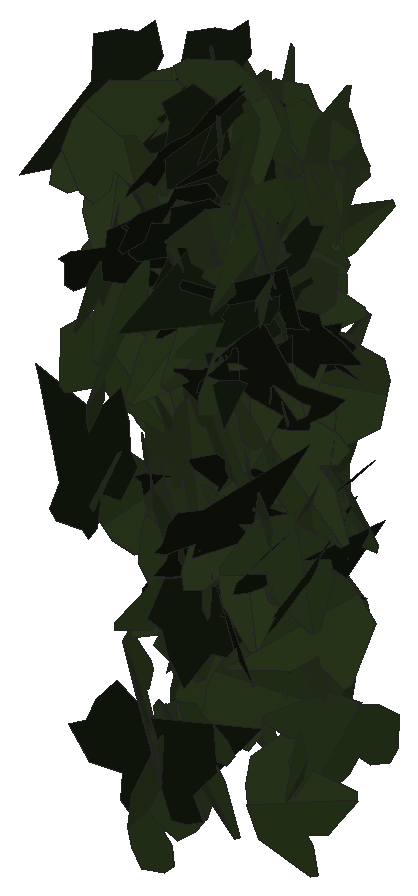
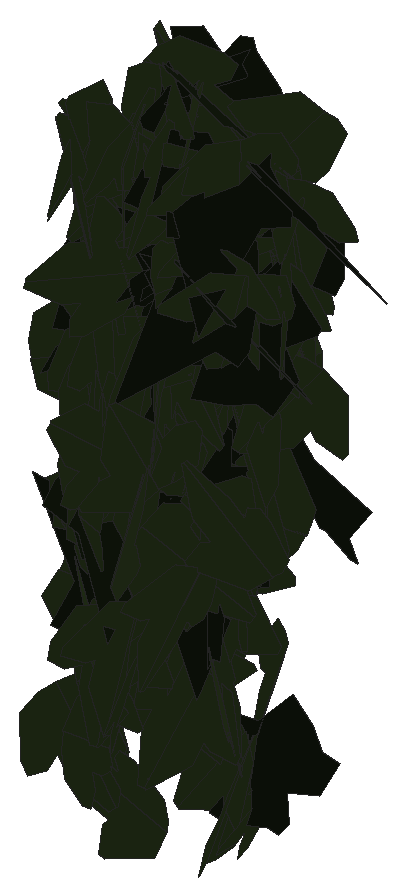
# SketchUp Ruby script. Lengths in inches.
U = 1.inch
M = Sketchup.active_model
def pt(a) = Geom::Point3d.new(a.map { |v| v * U })
def face(e, loops, mat)
  f = e.add_face(loops[0].map { |a| pt(a) })
  loops[1..].each { |l| e.add_face(l.map { |a| pt(a) }).erase! }
  f.material = f.back_material = mat if mat
  f
end
# faces: each face lists its corners as indices into pts; further lists are holes
def faces(e, pts, list, mat = nil) = list.each { |f| face(e, (f[0].is_a?(Array) ? f : [f]).map { |l| l.map { |i| pts[i] } }, mat) }
# xy, xz, yz: faces in a plane at the given z, y or x. An outline is a flat list of corners, or four numbers for a rectangle; further outlines are holes
def ring(l) = l.size == 4 ? [[l[0], l[1]], [l[2], l[1]], [l[2], l[3]], [l[0], l[3]]] : l.each_slice(2).to_a
def flat(e, list, mat, &to3) = list.each { |f| face(e, (f[0].is_a?(Array) ? f : [f]).map { |l| ring(l).map { |u, v| to3.(u, v) } }, mat) }
def xy(e, z, list, mat = nil) = flat(e, list, mat) { |x, y| [x, y, z] }
def xz(e, y, list, mat = nil) = flat(e, list, mat) { |x, z| [x, y, z] }
def yz(e, x, list, mat = nil) = flat(e, list, mat) { |y, z| [x, y, z] }
def lines(e, pts, list) = list.each { |a, b| e.add_line(pt(pts[a]), pt(pts[b])) }
# prism: a flat outline (further loops are holes) pulled along v
def prism(e, loops, v, mat = nil)
  f = face(e, loops, mat); d = Geom::Vector3d.new(v.map { |x| x * U })
  f.pushpull(f.normal.samedirection?(d) ? d.length : -d.length)
end
def box(e, o, s, mat = nil) = prism(e, [[o, [o[0] + s[0], o[1], o[2]], [o[0] + s[0], o[1] + s[1], o[2]], [o[0], o[1] + s[1], o[2]]]], [0, 0, s[2]], mat)
def at(x, y, z, deg = 0) = Geom::Transformation.translation(pt([x, y, z])) * Geom::Transformation.rotation(ORIGIN, Z_AXIS, deg.degrees)
def axes(o, x, y, z) = Geom::Transformation.new([*x, 0, *y, 0, *z, 0, *pt(o).to_a, 1])
def part(name) = M.definitions.add(name)
# library, detail: a bought-in or finely detailed component or shape, given as its bounding box
def library(name, o, s) = part(name).tap { |d| box(d.entities, o, s) }
def detail(e, o, s) = box(e.add_group.entities, o, s)
def put(e, d, t, mat = nil) = e.add_instance(d, t).tap { |i| i.material = mat if mat }
def group(e, t, mat = nil) = e.add_group.tap { |g| g.transformation = t; g.material = mat if mat }.entities
root = M.entities
M.materials.add("efeu1").color = [18, 25, 13]
M.materials.add("efeu2").color = [43, 57, 29]
c1 = part("ivyleaf_9")
p = [[1.54,2.16,1.25],[1.36,2.04,1.19],[-0.21,0.99,0.68],[-0.71,1.11,0.82],[-0.85,0.86,0.67],[-0.8,0.17,0.21],
  [-0.9,-0.01,0.1],[-0.67,-0.16,-0.02],[-0.08,-0.08,-0.05],[-0.03,-0.6,-0.4],[0.65,-0.88,-0.66],[0.83,-0.6,-0.49],
  [1.29,-0.42,-0.43],[1.8125,-0.07,-0.26],[1.21,0.44,0.15]]
faces(c1.entities,p,[[0,1,2,3,4,5,6,7,8,9,10,11,12,13,14]],"efeu1")
c2 = part("ivyleaf_10")
p = [[0,0.5,-0.03],[-0.0625,2.02,-0.43],[-0.19,2.01,-0.46],[-0.54,1.05,-0.29],[-0.52,0.625,-0.18],[-0.83,0.76,-0.28],
  [-1.16,0.64,-0.33],[-1.15,0.33,-0.24],[-0.77,-0.39,0.02],[-0.3,-0.51,0.16],[0.04,-0.48,0.23],[-0.02,2.01,-0.4375],
  [-0.06,2.01,-0.43],[0.04,-0.49,0.23],[0.67,-0.49,0.14],[1.38,0.36,-0.2],[1.375,0.51,-0.24],[0.81,0.65,-0.19],
  [0.62,0.59,-0.15],[0.6,1.09,-0.28],[0.5,1.23,-0.31]]
faces(c2.entities,p,[[0,1,2,3,4,5,6,7,8,9,10],[11,12,0,13,14,15,16,17,18,19,20]],"efeu2")
put(root,c1,axes([53.01,224.28,213.86],[-0.08194,0.49287,-0.01911],[0.00066,-0.01926,-0.49963],[-0.49324,-0.08191,0.00251]))
put(root,c2,axes([53.49,224.47,213.82],[0.29891,-0.37756,-0.13453],[-0.0781,0.10975,-0.48151],[0.39313,0.30888,0.00664]))
put(root,c2,axes([53.17,224.42,212.98],[-0.47923,-0.13524,-0.04522],[0.04223,0.01686,-0.49793],[0.13621,-0.48107,-0.00474]))
put(root,c1,axes([52.24,224.17,212.53],[0.31543,0.37494,0.09961],[0.06207,0.07795,-0.48997],[-0.38295,0.32147,0.00263]))
put(root,c2,axes([52.11,224.1875,211.125],[0.20626,-0.0813,0.44816],[-0.28646,0.35934,0.19702],[-0.35412,-0.33803,0.10166]))
put(root,c2,axes([52.12,224.58,213.11],[-0.31863,0.21038,-0.32282],[0.27616,-0.16744,-0.3817],[-0.26871,-0.42155,-0.00949]))
put(root,c2,axes([53.54,224.875,212.99],[0.00931,-0.29036,0.40695],[0.04826,-0.40459,-0.28978],[0.49758,0.04467,0.02049]))
put(root,c2,axes([52.0625,224.58,212.13],[0.44448,-0.22083,-0.06058],[-0.0461,0.04328,-0.49599],[0.2243,0.4465,0.01812]))
put(root,c2,axes([53.64,224.52,212.875],[0.3422,-0.33023,-0.15444],[-0.09926,0.11941,-0.47528],[0.35078,0.35594,0.01617]))
put(root,c1,axes([52.86,224.23,213.17],[0.13472,0.46802,0.11315],[0.03132,0.10873,-0.48703],[-0.48049,0.13832,-0.00002]))
put(root,c2,axes([53.26,224.81,212],[-0.22024,-0.24089,0.37877],[-0.18429,-0.33618,-0.32097],[0.4093,-0.28099,0.0593]))
put(root,c2,axes([53.59,224.49,213.13],[-0.30366,0.39692,0.01568],[-0.01009,0.01203,-0.49975],[-0.3971,-0.30383,0.0007]))
put(root,c1,axes([53,224.46,209.82],[0.24907,0.43347,0.00838],[-0.0061,-0.00616,0.49992],[0.4335,-0.24914,0.00222]))
put(root,c1,axes([53.27,224.6875,211.9],[0.494,0.07725,-0.00036],[-0.00038,0.00479,0.49998],[0.07725,-0.49397,0.00479]))
put(root,c1,axes([52.83,224.3125,212.89],[0.38483,0.31697,0.03793],[0.02521,0.02905,-0.49852],[-0.31824,0.3856,0.00638]))
put(root,c1,axes([53.42,224.87,212.58],[-0.42674,-0.15396,0.21021],[-0.1897,-0.09295,-0.45318],[0.17863,-0.46654,0.02092]))
put(root,c2,axes([52.18,224.59,208.21],[-0.29106,0.39887,-0.07866],[0.04703,-0.06305,-0.49377],[-0.40382,-0.29483,-0.00081]))
put(root,c2,axes([51.88,224.68,213.07],[0.49749,0.03328,0.03743],[0.03738,0.00194,-0.4986],[-0.03333,0.49889,-0.00056]))
put(root,c2,axes([52.03,224.375,213.56],[0.17565,0.3024,0.35735],[0.14418,0.32818,-0.34858],[-0.44537,0.2255,0.0281]))
put(root,c1,axes([51.91,224.42,209.96],[-0.05106,0.12132,0.48236],[-0.2897,0.38691,-0.12798],[-0.40431,-0.29255,0.03079]))
put(root,c2,axes([51.97,224.48,212.25],[0.05305,-0.37741,-0.32364],[-0.0349,0.32185,-0.38104],[0.49595,0.06302,0.0078]))
put(root,c1,axes([53.73,224.56,212.55],[-0.28381,0.35846,0.20238],[-0.2025,0.09244,-0.44772],[-0.35839,-0.3361,0.09271]))
put(root,c2,axes([53.65,224.83,212.46],[-0.2618,-0.37422,0.20353],[-0.11137,-0.17045,-0.45666],[0.41117,-0.28444,0.00589]))
put(root,c1,axes([53.21,224.81,211.06],[0.47177,0.10045,0.13169],[-0.12898,-0.02657,0.48235],[0.1039,-0.48908,0.00084]))
put(root,c2,axes([52.72,224.7,209.11],[-0.27081,-0.41819,-0.04217],[0.02998,0.03081,-0.49815],[0.41924,-0.27234,0.00839]))
put(root,c2,axes([52.9375,224.6875,211.05],[-0.45123,0.17443,-0.12635],[0.11304,-0.05787,-0.4836],[-0.18334,-0.465,0.01279]))
put(root,c2,axes([53.17,224.98,213.5],[0.16317,-0.39651,0.25721],[0.08733,-0.24212,-0.42866],[0.46449,0.18481,-0.00976]))
put(root,c2,axes([53.5,224.69,212.08],[-0.34925,0.18892,-0.30386],[-0.28043,0.11919,0.39642],[0.22222,0.44733,0.0227]))
put(root,c2,axes([52.4375,224.58,209.99],[-0.34802,0.20839,0.29233],[-0.26084,0.13298,-0.40532],[-0.24667,-0.43462,0.01615]))
put(root,c2,axes([53.26,224.84,211.88],[-0.15431,-0.47253,0.0539],[-0.00488,-0.05509,-0.49693],[0.47557,-0.15389,0.01239]))
put(root,c2,axes([51.73,224.76,211.22],[-0.38038,-0.133,-0.29601],[0.3159,-0.04738,-0.38465],[0.07426,-0.47965,0.12007]))
put(root,c2,axes([52.65,224.79,210.62],[-0.07809,0.48217,-0.10686],[0.01846,-0.10526,-0.48845],[-0.49352,-0.08023,-0.00136]))
put(root,c2,axes([52.85,224.68,212.46],[-0.42716,0.25307,0.05904],[-0.05057,0.03048,-0.4965],[-0.2549,-0.43015,-0.00044]))
put(root,c1,axes([51.98,224.74,207.09],[0.01906,0.00281,0.49963],[0.475,-0.15517,-0.01725],[0.15496,0.4753,-0.00858]))
put(root,c2,axes([53.13,224.84,213.93],[0.3117,-0.00481,-0.39092],[-0.39046,0.02115,-0.31159],[0.01953,0.49953,0.00943]))
put(root,c2,axes([52.72,224.92,212.78],[0.39517,-0.30034,0.06033],[0.04868,-0.03566,-0.49635],[0.30245,0.39815,0.00106]))
put(root,c2,axes([52.46,224.79,209.88],[-0.49592,-0.00803,-0.06327],[0.06366,-0.03258,-0.49486],[0.00382,-0.49887,0.03334]))
put(root,c1,axes([52.92,224.83,213.84],[0.10067,-0.42668,-0.24043],[-0.05798,0.23335,-0.43839],[0.48632,0.11615,-0.0025]))
put(root,c2,axes([53.3,224.79,211.54],[0.18564,0.46371,-0.02252],[-0.07708,0.00687,-0.49398],[-0.45782,0.18688,0.07403]))
put(root,c1,axes([53.54,224.66,212.07],[0.37316,0.26057,-0.20701],[-0.17134,-0.11621,-0.45513],[-0.2853,0.41061,0.00256]))
put(root,c2,axes([52.375,224.49,206.86],[-0.03378,0.02898,0.49802],[-0.2316,0.44119,-0.04138],[-0.44184,-0.23347,-0.01638]))
put(root,c1,axes([52.86,224.95,213.98],[-0.45968,0.19524,0.02403],[-0.05286,-0.06377,-0.49309],[-0.18948,-0.45587,0.07927]))
put(root,c1,axes([52.78,224.65,209.25],[0.18669,-0.19967,-0.41867],[-0.17703,0.38647,-0.26325],[0.42873,0.24652,0.07361]))
put(root,c2,axes([51.95,225.04,210.3],[-0.21238,0.08744,0.44413],[0.4188,-0.14818,0.22945],[0.17175,0.46947,-0.0103]))
put(root,c1,axes([52.91,225.13,212.2],[-0.08359,-0.49295,-0.00395],[-0.00256,0.00444,-0.49997],[0.49296,-0.08357,-0.00326]))
put(root,c1,axes([53.57,224.76,211.71],[0.11106,0.45314,-0.17981],[-0.04411,-0.17432,-0.46655],[-0.48551,0.11949,0.00125]))
put(root,c1,axes([52.5,224.7,211.73],[0.15435,0.47301,-0.0494],[0.0114,0.04824,0.49754],[0.47544,-0.15472,0.00411]))
put(root,c2,axes([52.55,224.89,209.47],[0.41459,-0.23711,-0.14797],[-0.0927,0.13307,-0.47297],[0.26367,0.41961,0.06638]))
put(root,c2,axes([52.52,225.08,211.63],[0.31116,0.25764,-0.29462],[-0.22707,-0.18771,-0.40398],[-0.31877,0.38521,0.00019]))
put(root,c2,axes([52.07,224.67,209.67],[-0.07449,-0.25388,0.42426],[0.10852,0.41019,0.26451],[-0.48236,0.13149,-0.006]))
put(root,c2,axes([52.67,225.2,213.45],[-0.15396,0.13151,0.45717],[0.34143,-0.30404,0.20244],[0.33124,0.37452,0.00382]))
put(root,c2,axes([53.03,224.89,210.41],[-0.393,0.30877,-0.01441],[0.01315,-0.00659,-0.49978],[-0.30883,-0.39321,-0.00294]))
put(root,c1,axes([52.65,224.85,213.04],[-0.16412,0.46431,-0.08649],[0.0358,-0.07908,-0.49241],[-0.47094,-0.16782,-0.00729]))
put(root,c2,axes([53.07,224.93,209.68],[0.3105,0.38869,0.05014],[0.03982,0.03234,-0.49736],[-0.38988,0.31285,-0.01087]))
put(root,c2,axes([53.5,224.91,212.01],[-0.14452,-0.45659,-0.14367],[0.05417,0.13351,-0.47879],[0.47558,-0.15395,0.01088]))
put(root,c2,axes([52.66,225.33,212.22],[-0.03982,-0.04274,-0.49658],[-0.32404,-0.37628,0.05837],[-0.3787,0.32647,0.00227]))
put(root,c2,axes([53.1,224.9,210.12],[-0.31693,0.07908,0.37855],[-0.37631,0.04973,-0.32545],[-0.08912,-0.4912,0.02799]))
put(root,c2,axes([52.96,224.99,213.45],[-0.44849,-0.21192,0.06286],[-0.06107,-0.01784,-0.49594],[0.21244,-0.45252,-0.00988]))
put(root,c2,axes([52.37,225.03,207.5],[-0.37722,0.1978,-0.26189],[0.2342,-0.11727,-0.42591],[-0.22991,-0.44399,-0.00418]))
put(root,c2,axes([53.52,224.91,212.05],[0.27366,0.40682,0.09801],[0.00926,0.11119,-0.48739],[-0.41836,0.26857,0.05333]))
put(root,c1,axes([52.37,225.21,209.11],[0.09274,-0.00533,-0.49129],[0.49021,-0.03268,0.09289],[-0.03311,-0.4989,-0.00084]))
put(root,c1,axes([53.19,224.82,211.93],[0.48815,0.08961,0.06063],[0.05117,0.05563,-0.49425],[-0.09533,0.48875,0.04515]))
put(root,c2,axes([53.49,224.73,212.96],[0.16045,0.25928,0.39627],[0.05579,0.40513,-0.28767],[-0.47026,0.13653,0.10108]))
put(root,c2,axes([52.8,225.2,208.2],[-0.38575,-0.20421,0.24391],[-0.15389,-0.21574,-0.424],[0.27841,-0.40219,0.10359]))
put(root,c1,axes([52.5625,224.8,210.11],[0.41487,0.27602,0.04118],[0.0249,0.03687,-0.49802],[-0.27796,0.41527,0.01685]))
put(root,c2,axes([52.375,224.76,209.57],[-0.01688,0.35307,0.35364],[-0.0577,0.3501,-0.35228],[-0.49637,-0.0527,0.02892]))
put(root,c2,axes([53.27,225.27,212.06],[0.2908,-0.34354,0.21775],[0.1677,-0.1426,-0.44894],[0.37056,0.33414,0.03228]))
put(root,c2,axes([53.3,225.11,210.56],[-0.37831,-0.06591,-0.32021],[0.3269,-0.08189,-0.36936],[-0.00375,-0.48883,0.10505]))
put(root,c2,axes([53.52,225.12,209.77],[-0.30071,-0.3952,-0.0582],[0.10175,-0.00534,-0.48951],[0.38629,-0.30625,0.08364]))
put(root,c1,axes([51.75,225.19,213.44],[-0.47635,0.14666,0.03981],[-0.04242,-0.00255,-0.49819],[-0.14592,-0.478,0.01488]))
put(root,c1,axes([52.73,224.92,209.46],[0.07893,0.48998,-0.06075],[-0.01152,-0.05968,-0.49629],[-0.4936,0.07974,0.00187]))
put(root,c2,axes([53.24,225.42,209.77],[-0.10932,0.26333,0.41074],[0.04379,-0.41393,0.27703],[0.48593,0.09654,0.06744]))
put(root,c2,axes([53,225.02,211.23],[-0.22421,0.03012,0.4459],[-0.4423,0.05658,-0.22622],[-0.06408,-0.49587,0.00127]))
put(root,c2,axes([52.34,225.08,212.71],[0.07927,0.49358,0.00999],[-0.00128,0.01032,-0.49989],[-0.49367,0.07923,0.0029]))
put(root,c2,axes([53.08,225.12,213.87],[-0.44643,0.17716,0.13898],[-0.17421,-0.07624,-0.46243],[-0.14266,-0.4613,0.1298]))
put(root,c2,axes([52.15,225.12,213.54],[0.26695,0.42271,-0.00749],[-0.02526,0.0071,-0.49931],[-0.42202,0.26696,0.02515]))
put(root,c1,axes([51.81,224.98,211.73],[0.29458,0.35422,-0.1943],[0.12744,0.14672,0.46069],[0.38338,-0.32094,-0.00384]))
put(root,c2,axes([52.4,225.18,208.87],[-0.28483,-0.38729,-0.13741],[0.2208,-0.00322,-0.44859],[0.34658,-0.31623,0.17286]))
put(root,c2,axes([52.38,225.14,213.32],[0.12089,0.48503,0.01166],[0.00059,0.01187,-0.49986],[-0.48517,0.12087,0.00229]))
put(root,c2,axes([53.66,225.41,208.94],[0.17068,0.17341,-0.4368],[-0.36064,-0.24965,-0.24003],[-0.30134,0.39699,0.03986]))
put(root,c1,axes([52.48,225.26,212.27],[-0.43882,0.23904,0.01729],[-0.03801,-0.03381,-0.49741],[-0.23663,-0.43785,0.04784]))
put(root,c2,axes([53.33,225.45,210.01],[-0.28392,-0.17591,0.37209],[-0.22375,-0.31342,-0.31891],[0.34544,-0.3476,0.09925]))
put(root,c2,axes([52.25,225.26,206.7],[-0.15372,0.46871,0.08172],[0.01975,-0.07951,0.49324],[0.47537,0.15487,0.00593]))
put(root,c2,axes([52.19,225.34,208.4375],[0.25018,-0.43106,0.03995],[0.03686,-0.02477,-0.49802],[0.43134,0.25214,0.01939]))
put(root,c1,axes([53.67,225.2,209.54],[-0.30081,0.39823,-0.03049],[0.0163,-0.02589,-0.49906],[-0.39906,-0.30124,0.0026]))
put(root,c2,axes([52.13,225.34,212.53],[0.47508,-0.14707,-0.05171],[-0.04679,0.02371,-0.49724],[0.14871,0.47729,0.00876]))
put(root,c2,axes([53.88,225.47,211.14],[-0.06963,-0.02411,-0.49454],[-0.46727,-0.16195,0.07368],[-0.16373,0.47243,0.00002]))
put(root,c2,axes([53.11,225.45,213.61],[0.00776,0.43919,-0.23886],[0.00189,-0.23892,-0.43922],[-0.49994,0.00591,-0.00537]))
put(root,c2,axes([53.42,225.27,211.3],[-0.12734,-0.46126,-0.145],[0.02857,0.14251,-0.47841],[0.48267,-0.13013,-0.00993]))
put(root,c1,axes([52.31,225.16,213.38],[0.29468,0.36575,-0.17143],[-0.11103,-0.13068,-0.46967],[-0.38838,0.31488,0.0042]))
put(root,c2,axes([52.66,225.55,209.63],[-0.20119,-0.23725,0.39145],[-0.2591,-0.29347,-0.31103],[0.37735,-0.328,-0.00486]))
put(root,c1,axes([53.14,225.22,208.86],[0.28694,0.40757,-0.03936],[0.0054,0.04429,0.498],[0.40943,-0.28622,0.02102]))
put(root,c2,axes([53.18,225.31,210.36],[-0.49903,-0.01574,0.02683],[-0.02661,-0.00713,-0.49924],[0.0161,-0.4997,0.00628]))
put(root,c2,axes([53.23,225.34,213.41],[0.3855,0.11048,0.29863],[0.28178,0.09999,-0.40075],[-0.14827,0.47728,0.01483]))
put(root,c2,axes([52.34,225.15,213.09],[0.1621,0.14774,0.44933],[0.29663,0.33822,-0.21822],[-0.36842,0.33732,0.022]))
put(root,c2,axes([53.34,225.44,211.375],[-0.41567,-0.27306,0.05153],[-0.01714,-0.06736,-0.49515],[0.27735,-0.4134,0.04664]))
put(root,c2,axes([53.45,225.59,211.08],[-0.03366,-0.4707,0.16524],[0.04312,-0.16774,-0.46905],[0.497,-0.01733,0.05188]))
put(root,c2,axes([52.94,225.09,208.12],[0.1887,0.12354,0.44624],[0.1515,0.43887,-0.18557],[-0.43754,0.20525,0.1282]))
put(root,c2,axes([53.14,225.1875,210.97],[-0.1835,0.39573,0.24438],[-0.12558,0.2108,-0.43565],[-0.44783,-0.22127,0.02203]))
put(root,c2,axes([53.48,225.8,210.02],[-0.02742,-0.03679,-0.49789],[0.03225,-0.49773,0.035],[-0.4982,-0.0302,0.02967]))
put(root,c2,axes([52.96,225.49,206.8],[0.16449,-0.03884,-0.47057],[0.45177,-0.13193,0.16881],[-0.13727,-0.48071,-0.00831]))
put(root,c2,axes([52.5,225.38,208.12],[-0.47313,-0.03373,-0.15813],[0.15804,0.00692,-0.47432],[0.03419,-0.49881,0.00411]))
put(root,c2,axes([51.93,225.39,212.37],[0.28095,0.40414,0.08798],[0.0477,0.07399,-0.49219],[-0.41084,0.28495,0.00302]))
put(root,c2,axes([53.17,225.34,211.33],[-0.24051,0.42853,0.09231],[-0.08031,0.06043,-0.48979],[-0.43094,-0.25043,0.03976]))
put(root,c1,axes([52.21,225.31,212.35],[0.48777,0.10913,-0.01292],[-0.01298,-0.00113,-0.49983],[-0.10912,0.48794,0.00173]))
put(root,c2,axes([52.79,225.25,213.38],[0.00196,-0.29779,-0.40165],[0.02681,0.40113,-0.29727],[0.49928,-0.02037,0.01754]))
put(root,c2,axes([53.63,225.6875,207.72],[-0.27969,-0.36083,0.2039],[-0.11412,-0.16943,-0.45637],[0.39844,-0.30182,0.01242]))
put(root,c2,axes([52.84,225.31,211.24],[0.14207,-0.24582,-0.41157],[-0.11153,0.40054,-0.27773],[0.46624,0.17072,0.05897]))
put(root,c2,axes([53.71,225.22,213.4],[-0.09592,0.21038,0.44333],[-0.19459,0.39838,-0.23115],[-0.45048,-0.21688,0.00545]))
put(root,c1,axes([53.4,225.31,209.73],[-0.00311,0.475,0.15609],[-0.05745,0.15472,-0.47197],[-0.49668,-0.02088,0.05362]))
put(root,c2,axes([53.16,225.8,208.32],[0.25539,-0.33018,-0.27523],[0.17252,-0.2145,0.41741],[-0.39372,-0.30817,0.00437]))
put(root,c2,axes([53.24,225.99,207.7],[0.06196,-0.26481,0.41957],[0.17118,-0.38546,-0.26855],[0.46568,0.17692,0.04289]))
put(root,c2,axes([53.57,225.46,210.76],[0.23133,-0.24168,-0.37159],[-0.17246,0.33705,-0.32658],[0.40834,0.27927,0.07258]))
put(root,c2,axes([53.74,225.55,213.32],[0.24549,-0.30249,-0.31342],[-0.18817,0.25082,-0.38946],[0.39284,0.30918,0.00931]))
put(root,c2,axes([53.21,225.87,209.83],[0.01137,-0.06164,0.49606],[0.48704,-0.11032,-0.02487],[0.11252,0.48377,0.05754]))
put(root,c2,axes([53.15,225.4375,213.24],[-0.09515,0.2157,-0.44093],[-0.15789,0.41182,0.23553],[0.46477,0.18406,-0.01026]))
put(root,c2,axes([51.49,225.77,210.05],[0.37588,-0.01386,-0.32942],[0.32825,-0.03133,0.37586],[-0.03106,-0.49882,-0.01445]))
put(root,c2,axes([52.875,225.84,209.55],[-0.31862,0.38256,0.04613],[0.02683,-0.03769,0.49786],[0.3844,0.31973,0.00349]))
put(root,c2,axes([53.26,225.49,212.16],[0.04384,-0.15532,0.47324],[0.00693,0.47521,0.15532],[-0.49803,-0.00706,0.04382]))
put(root,c2,axes([52.71,225.65,210.39],[0.22746,0.37023,-0.24736],[0.13642,0.20646,0.43447],[0.42385,-0.26514,-0.00709]))
put(root,c2,axes([52.91,225.95,208.8125],[-0.49748,-0.05009,-0.00007],[0.00006,0.00002,-0.5],[0.05009,-0.49748,-0.00001]))
put(root,c2,axes([53.11,225.78,210.5],[0.08275,-0.33151,0.36504],[-0.09507,0.35247,0.34165],[-0.48385,-0.12595,-0.0047]))
put(root,c2,axes([53.11,225.94,208.42],[-0.31995,0.14392,-0.35626],[-0.32123,0.15416,0.35078],[0.21081,0.45334,-0.00619]))
put(root,c2,axes([52.67,226.01,208.625],[-0.23212,0.43539,-0.08094],[0.03372,-0.07375,-0.49338],[-0.44157,-0.23451,0.00488]))
put(root,c2,axes([52.17,225.85,209.51],[0.02593,0.45581,0.20388],[0.00121,0.2041,-0.45645],[-0.49933,0.02416,0.00948]))
put(root,c2,axes([52.7,225.98,209.01],[0.09181,0.46755,0.15156],[-0.08054,0.1664,-0.46457],[-0.48485,0.06089,0.10587]))
